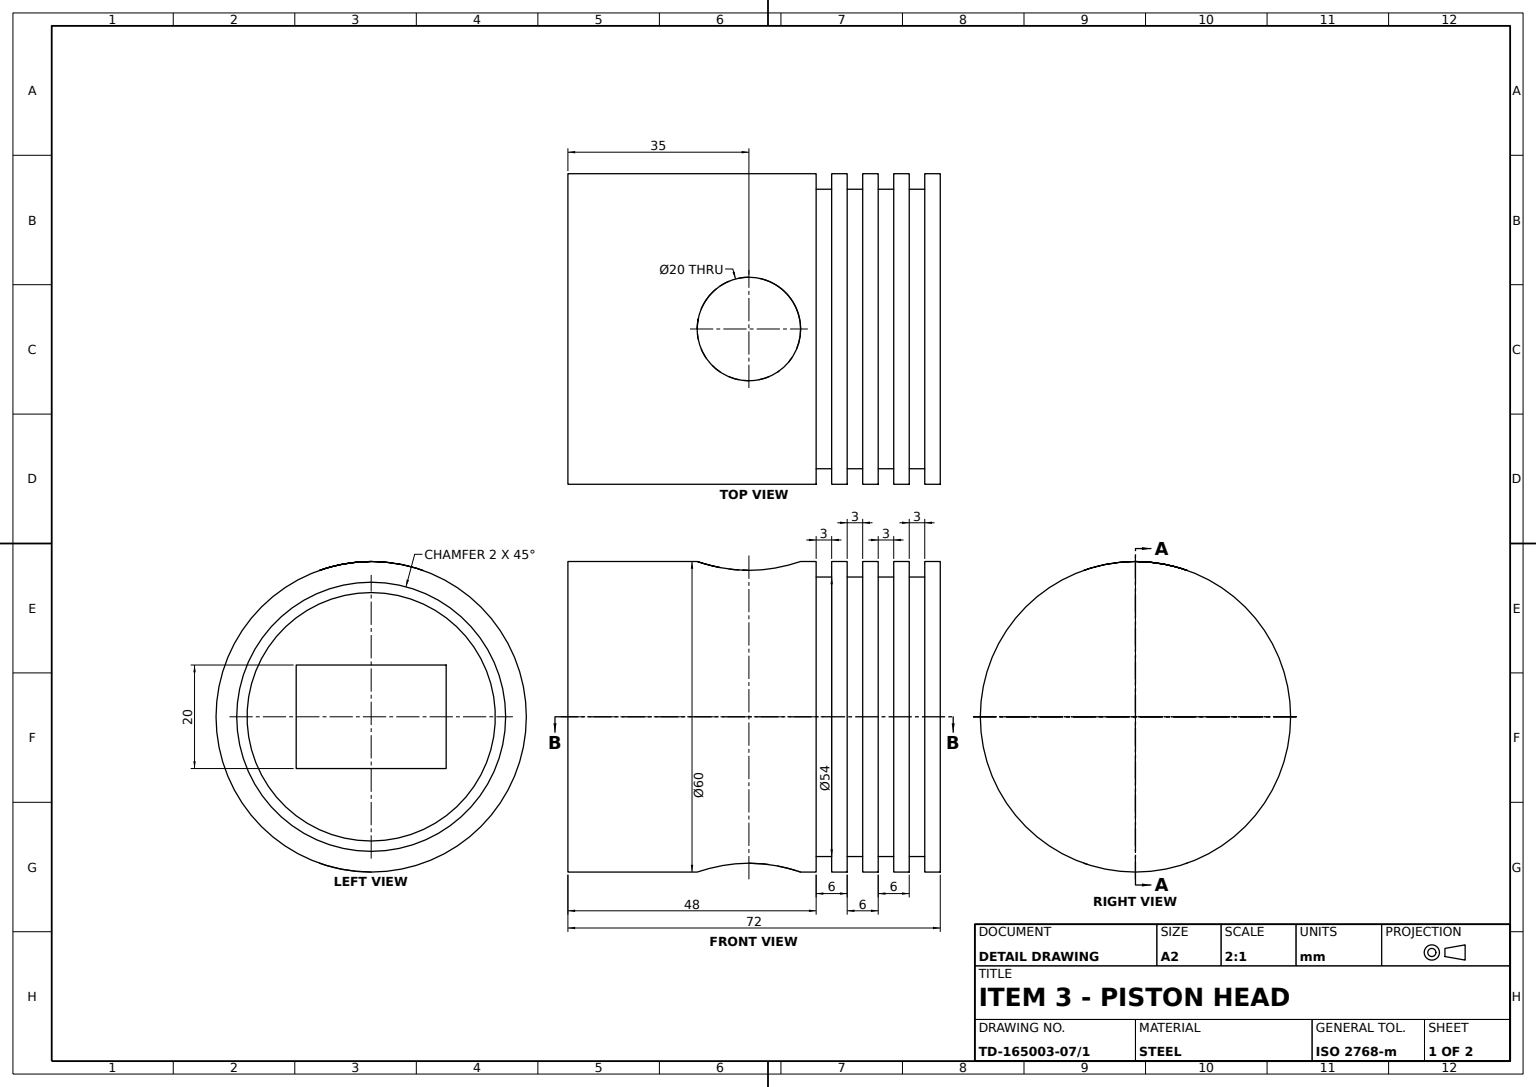
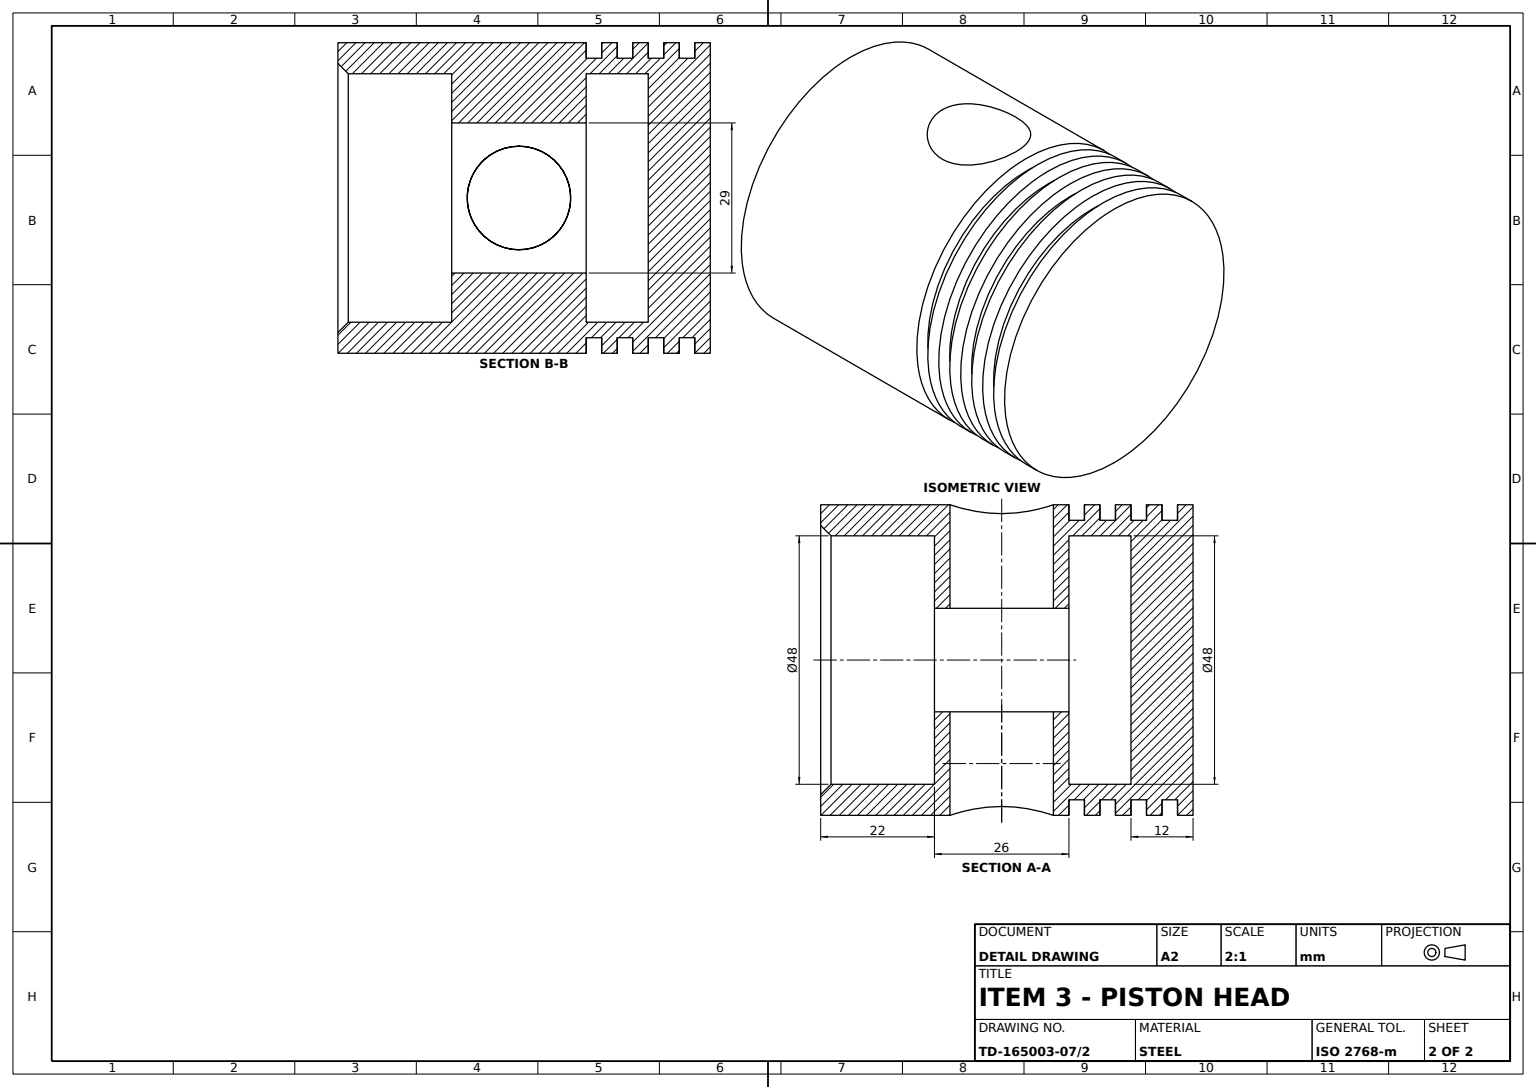
ISO-10303-21;
HEADER;
FILE_DESCRIPTION((''),'2;1');
FILE_NAME('','',(''),(''),'','','');
FILE_SCHEMA(('AUTOMOTIVE_DESIGN'));
ENDSEC;
DATA;
#1=APPLICATION_CONTEXT('');
#2=PRODUCT_CONTEXT('',#1,'mechanical');
#3=PRODUCT('','','',(#2));
#4=PRODUCT_DEFINITION_FORMATION('','',#3);
#5=PRODUCT_DEFINITION_CONTEXT('',#1,'design');
#6=PRODUCT_DEFINITION('','',#4,#5);
#7=PRODUCT_DEFINITION_SHAPE('','',#6);
#8=(LENGTH_UNIT()NAMED_UNIT(*)SI_UNIT(.MILLI.,.METRE.));
#9=(NAMED_UNIT(*)PLANE_ANGLE_UNIT()SI_UNIT($,.RADIAN.));
#10=(NAMED_UNIT(*)SI_UNIT($,.STERADIAN.)SOLID_ANGLE_UNIT());
#11=UNCERTAINTY_MEASURE_WITH_UNIT(LENGTH_MEASURE(1.E-05),#8,'distance_accuracy_value','');
#12=(GEOMETRIC_REPRESENTATION_CONTEXT(3)GLOBAL_UNCERTAINTY_ASSIGNED_CONTEXT((#11))GLOBAL_UNIT_ASSIGNED_CONTEXT((#8,#9,#10))REPRESENTATION_CONTEXT('',''));
#13=CARTESIAN_POINT('',(27.,51.,0.));
#14=VERTEX_POINT('',#13);
#15=CARTESIAN_POINT('',(27.,48.,0.));
#16=VERTEX_POINT('',#15);
#17=CARTESIAN_POINT('',(27.,60.,0.));
#18=DIRECTION('',(0.,-1.,0.));
#19=VECTOR('',#18,1000.);
#20=LINE('',#17,#19);
#21=EDGE_CURVE('',#14,#16,#20,.T.);
#22=ORIENTED_EDGE('',*,*,#21,.T.);
#23=CARTESIAN_POINT('',(-27.,48.,0.));
#24=VERTEX_POINT('',#23);
#25=CARTESIAN_POINT('',(0.,48.,0.));
#26=DIRECTION('',(1.,0.,0.));
#27=AXIS2_PLACEMENT_3D('',#25,#18,#26);
#28=CIRCLE('',#27,27.);
#29=EDGE_CURVE('',#24,#16,#28,.T.);
#30=ORIENTED_EDGE('',*,*,#29,.F.);
#31=CARTESIAN_POINT('',(-27.,51.,0.));
#32=VERTEX_POINT('',#31);
#33=CARTESIAN_POINT('',(-27.,60.,0.));
#34=LINE('',#33,#19);
#35=EDGE_CURVE('',#32,#24,#34,.T.);
#36=ORIENTED_EDGE('',*,*,#35,.F.);
#37=CARTESIAN_POINT('',(0.,51.,0.));
#38=AXIS2_PLACEMENT_3D('',#37,#18,#26);
#39=CIRCLE('',#38,27.);
#40=EDGE_CURVE('',#32,#14,#39,.T.);
#41=ORIENTED_EDGE('',*,*,#40,.T.);
#42=EDGE_LOOP('',(#22,#30,#36,#41));
#43=FACE_OUTER_BOUND('',#42,.T.);
#44=CARTESIAN_POINT('',(0.,60.,0.));
#45=AXIS2_PLACEMENT_3D('',#44,#18,#26);
#46=CYLINDRICAL_SURFACE('',#45,27.);
#47=ADVANCED_FACE('',(#43),#46,.T.);
#48=CARTESIAN_POINT('',(27.,69.,0.));
#49=VERTEX_POINT('',#48);
#50=CARTESIAN_POINT('',(-27.,69.,0.));
#51=VERTEX_POINT('',#50);
#52=CARTESIAN_POINT('',(0.,69.,0.));
#53=AXIS2_PLACEMENT_3D('',#52,#18,#26);
#54=CIRCLE('',#53,27.);
#55=EDGE_CURVE('',#49,#51,#54,.T.);
#56=ORIENTED_EDGE('',*,*,#55,.T.);
#57=CARTESIAN_POINT('',(-27.,66.,0.));
#58=VERTEX_POINT('',#57);
#59=EDGE_CURVE('',#51,#58,#34,.T.);
#60=ORIENTED_EDGE('',*,*,#59,.T.);
#61=CARTESIAN_POINT('',(27.,66.,0.));
#62=VERTEX_POINT('',#61);
#63=CARTESIAN_POINT('',(0.,66.,0.));
#64=AXIS2_PLACEMENT_3D('',#63,#18,#26);
#65=CIRCLE('',#64,27.);
#66=EDGE_CURVE('',#62,#58,#65,.T.);
#67=ORIENTED_EDGE('',*,*,#66,.F.);
#68=EDGE_CURVE('',#49,#62,#20,.T.);
#69=ORIENTED_EDGE('',*,*,#68,.F.);
#70=EDGE_LOOP('',(#56,#60,#67,#69));
#71=FACE_OUTER_BOUND('',#70,.T.);
#72=ADVANCED_FACE('',(#71),#46,.T.);
#73=CARTESIAN_POINT('',(-30.,54.,0.));
#74=VERTEX_POINT('',#73);
#75=CARTESIAN_POINT('',(-30.,51.,0.));
#76=VERTEX_POINT('',#75);
#77=CARTESIAN_POINT('',(-30.,60.,0.));
#78=LINE('',#77,#19);
#79=EDGE_CURVE('',#74,#76,#78,.T.);
#80=ORIENTED_EDGE('',*,*,#79,.T.);
#81=CARTESIAN_POINT('',(30.,51.,0.));
#82=VERTEX_POINT('',#81);
#83=CIRCLE('',#38,30.);
#84=EDGE_CURVE('',#82,#76,#83,.T.);
#85=ORIENTED_EDGE('',*,*,#84,.F.);
#86=CARTESIAN_POINT('',(30.,54.,0.));
#87=VERTEX_POINT('',#86);
#88=CARTESIAN_POINT('',(30.,60.,0.));
#89=LINE('',#88,#19);
#90=EDGE_CURVE('',#87,#82,#89,.T.);
#91=ORIENTED_EDGE('',*,*,#90,.F.);
#92=CARTESIAN_POINT('',(0.,54.,0.));
#93=AXIS2_PLACEMENT_3D('',#92,#18,#26);
#94=CIRCLE('',#93,30.);
#95=EDGE_CURVE('',#87,#74,#94,.T.);
#96=ORIENTED_EDGE('',*,*,#95,.T.);
#97=EDGE_LOOP('',(#80,#85,#91,#96));
#98=FACE_OUTER_BOUND('',#97,.T.);
#99=CYLINDRICAL_SURFACE('',#45,30.);
#100=ADVANCED_FACE('',(#98),#99,.T.);
#101=CARTESIAN_POINT('',(30.,48.,0.));
#102=VERTEX_POINT('',#101);
#103=CARTESIAN_POINT('',(-30.,48.,0.));
#104=VERTEX_POINT('',#103);
#105=CIRCLE('',#27,30.);
#106=EDGE_CURVE('',#102,#104,#105,.T.);
#107=ORIENTED_EDGE('',*,*,#106,.F.);
#108=EDGE_CURVE('',#104,#102,#105,.T.);
#109=ORIENTED_EDGE('',*,*,#108,.F.);
#110=EDGE_LOOP('',(#107,#109));
#111=FACE_OUTER_BOUND('',#110,.T.);
#112=EDGE_CURVE('',#16,#24,#28,.T.);
#113=ORIENTED_EDGE('',*,*,#112,.T.);
#114=ORIENTED_EDGE('',*,*,#29,.T.);
#115=EDGE_LOOP('',(#113,#114));
#116=FACE_BOUND('',#115,.T.);
#117=AXIS2_PLACEMENT_3D('',#103,#18,#26);
#118=PLANE('',#117);
#119=ADVANCED_FACE('',(#111,#116),#118,.F.);
#120=VERTEX_POINT('',#77);
#121=VERTEX_POINT('',#88);
#122=CIRCLE('',#45,30.);
#123=EDGE_CURVE('',#120,#121,#122,.T.);
#124=ORIENTED_EDGE('',*,*,#123,.F.);
#125=EDGE_CURVE('',#121,#120,#122,.T.);
#126=ORIENTED_EDGE('',*,*,#125,.F.);
#127=EDGE_LOOP('',(#124,#126));
#128=FACE_OUTER_BOUND('',#127,.T.);
#129=VERTEX_POINT('',#33);
#130=VERTEX_POINT('',#17);
#131=CIRCLE('',#45,27.);
#132=EDGE_CURVE('',#129,#130,#131,.T.);
#133=ORIENTED_EDGE('',*,*,#132,.T.);
#134=EDGE_CURVE('',#130,#129,#131,.T.);
#135=ORIENTED_EDGE('',*,*,#134,.T.);
#136=EDGE_LOOP('',(#133,#135));
#137=FACE_BOUND('',#136,.T.);
#138=AXIS2_PLACEMENT_3D('',#77,#18,#26);
#139=PLANE('',#138);
#140=ADVANCED_FACE('',(#128,#137),#139,.F.);
#141=CARTESIAN_POINT('',(-30.,66.,0.));
#142=VERTEX_POINT('',#141);
#143=CARTESIAN_POINT('',(30.,66.,0.));
#144=VERTEX_POINT('',#143);
#145=CIRCLE('',#64,30.);
#146=EDGE_CURVE('',#142,#144,#145,.T.);
#147=ORIENTED_EDGE('',*,*,#146,.T.);
#148=CARTESIAN_POINT('',(30.,63.,0.));
#149=VERTEX_POINT('',#148);
#150=EDGE_CURVE('',#144,#149,#89,.T.);
#151=ORIENTED_EDGE('',*,*,#150,.T.);
#152=CARTESIAN_POINT('',(-30.,63.,0.));
#153=VERTEX_POINT('',#152);
#154=CARTESIAN_POINT('',(0.,63.,0.));
#155=AXIS2_PLACEMENT_3D('',#154,#18,#26);
#156=CIRCLE('',#155,30.);
#157=EDGE_CURVE('',#153,#149,#156,.T.);
#158=ORIENTED_EDGE('',*,*,#157,.F.);
#159=EDGE_CURVE('',#142,#153,#78,.T.);
#160=ORIENTED_EDGE('',*,*,#159,.F.);
#161=EDGE_LOOP('',(#147,#151,#158,#160));
#162=FACE_OUTER_BOUND('',#161,.T.);
#163=ADVANCED_FACE('',(#162),#99,.T.);
#164=CARTESIAN_POINT('',(-27.,63.,0.));
#165=VERTEX_POINT('',#164);
#166=EDGE_CURVE('',#165,#129,#34,.T.);
#167=ORIENTED_EDGE('',*,*,#166,.F.);
#168=CARTESIAN_POINT('',(27.,63.,0.));
#169=VERTEX_POINT('',#168);
#170=CIRCLE('',#155,27.);
#171=EDGE_CURVE('',#165,#169,#170,.T.);
#172=ORIENTED_EDGE('',*,*,#171,.T.);
#173=EDGE_CURVE('',#169,#130,#20,.T.);
#174=ORIENTED_EDGE('',*,*,#173,.T.);
#175=ORIENTED_EDGE('',*,*,#132,.F.);
#176=EDGE_LOOP('',(#167,#172,#174,#175));
#177=FACE_OUTER_BOUND('',#176,.T.);
#178=ADVANCED_FACE('',(#177),#46,.T.);
#179=CARTESIAN_POINT('',(24.,2.,0.));
#180=VERTEX_POINT('',#179);
#181=CARTESIAN_POINT('',(26.,0.,0.));
#182=VERTEX_POINT('',#181);
#183=DIRECTION('',(0.707106781,-0.707106781,0.));
#184=VECTOR('',#183,1000.);
#185=LINE('',#179,#184);
#186=EDGE_CURVE('',#180,#182,#185,.T.);
#187=ORIENTED_EDGE('',*,*,#186,.F.);
#188=CARTESIAN_POINT('',(-24.,2.,0.));
#189=VERTEX_POINT('',#188);
#190=CARTESIAN_POINT('',(0.,2.,0.));
#191=DIRECTION('',(-1.,0.,0.));
#192=AXIS2_PLACEMENT_3D('',#190,#18,#191);
#193=CIRCLE('',#192,24.);
#194=EDGE_CURVE('',#189,#180,#193,.T.);
#195=ORIENTED_EDGE('',*,*,#194,.F.);
#196=CARTESIAN_POINT('',(-26.,0.,0.));
#197=VERTEX_POINT('',#196);
#198=DIRECTION('',(-0.707106781,-0.707106781,0.));
#199=VECTOR('',#198,1000.);
#200=LINE('',#188,#199);
#201=EDGE_CURVE('',#189,#197,#200,.T.);
#202=ORIENTED_EDGE('',*,*,#201,.T.);
#203=CARTESIAN_POINT('',(0.,0.,0.));
#204=DIRECTION('',(0.,1.,0.));
#205=AXIS2_PLACEMENT_3D('',#203,#204,#191);
#206=CIRCLE('',#205,26.);
#207=EDGE_CURVE('',#182,#197,#206,.T.);
#208=ORIENTED_EDGE('',*,*,#207,.F.);
#209=EDGE_LOOP('',(#187,#195,#202,#208));
#210=FACE_OUTER_BOUND('',#209,.T.);
#211=AXIS2_PLACEMENT_3D('',#190,#18,#26);
#212=CONICAL_SURFACE('',#211,24.,0.785398163);
#213=ADVANCED_FACE('',(#210),#212,.F.);
#214=CARTESIAN_POINT('',(-27.,54.,0.));
#215=VERTEX_POINT('',#214);
#216=CARTESIAN_POINT('',(27.,54.,0.));
#217=VERTEX_POINT('',#216);
#218=CIRCLE('',#93,27.);
#219=EDGE_CURVE('',#215,#217,#218,.T.);
#220=ORIENTED_EDGE('',*,*,#219,.T.);
#221=EDGE_CURVE('',#217,#215,#218,.T.);
#222=ORIENTED_EDGE('',*,*,#221,.T.);
#223=EDGE_LOOP('',(#220,#222));
#224=FACE_BOUND('',#223,.T.);
#225=ORIENTED_EDGE('',*,*,#95,.F.);
#226=EDGE_CURVE('',#74,#87,#94,.T.);
#227=ORIENTED_EDGE('',*,*,#226,.F.);
#228=EDGE_LOOP('',(#225,#227));
#229=FACE_OUTER_BOUND('',#228,.T.);
#230=AXIS2_PLACEMENT_3D('',#73,#18,#26);
#231=PLANE('',#230);
#232=ADVANCED_FACE('',(#224,#229),#231,.F.);
#233=CARTESIAN_POINT('',(30.,72.,0.));
#234=VERTEX_POINT('',#233);
#235=CARTESIAN_POINT('',(30.,69.,0.));
#236=VERTEX_POINT('',#235);
#237=EDGE_CURVE('',#234,#236,#89,.T.);
#238=ORIENTED_EDGE('',*,*,#237,.F.);
#239=CARTESIAN_POINT('',(-30.,72.,0.));
#240=VERTEX_POINT('',#239);
#241=CARTESIAN_POINT('',(0.,72.,0.));
#242=AXIS2_PLACEMENT_3D('',#241,#18,#26);
#243=CIRCLE('',#242,30.);
#244=EDGE_CURVE('',#234,#240,#243,.T.);
#245=ORIENTED_EDGE('',*,*,#244,.T.);
#246=CARTESIAN_POINT('',(-30.,69.,0.));
#247=VERTEX_POINT('',#246);
#248=EDGE_CURVE('',#240,#247,#78,.T.);
#249=ORIENTED_EDGE('',*,*,#248,.T.);
#250=CIRCLE('',#53,30.);
#251=EDGE_CURVE('',#236,#247,#250,.T.);
#252=ORIENTED_EDGE('',*,*,#251,.F.);
#253=EDGE_LOOP('',(#238,#245,#249,#252));
#254=FACE_OUTER_BOUND('',#253,.T.);
#255=ADVANCED_FACE('',(#254),#99,.T.);
#256=ORIENTED_EDGE('',*,*,#84,.T.);
#257=EDGE_CURVE('',#76,#82,#83,.T.);
#258=ORIENTED_EDGE('',*,*,#257,.T.);
#259=EDGE_LOOP('',(#256,#258));
#260=FACE_OUTER_BOUND('',#259,.T.);
#261=ORIENTED_EDGE('',*,*,#40,.F.);
#262=EDGE_CURVE('',#14,#32,#39,.T.);
#263=ORIENTED_EDGE('',*,*,#262,.F.);
#264=EDGE_LOOP('',(#261,#263));
#265=FACE_BOUND('',#264,.T.);
#266=AXIS2_PLACEMENT_3D('',#31,#204,#191);
#267=PLANE('',#266);
#268=ADVANCED_FACE('',(#260,#265),#267,.F.);
#269=ORIENTED_EDGE('',*,*,#112,.F.);
#270=ORIENTED_EDGE('',*,*,#21,.F.);
#271=ORIENTED_EDGE('',*,*,#262,.T.);
#272=ORIENTED_EDGE('',*,*,#35,.T.);
#273=EDGE_LOOP('',(#269,#270,#271,#272));
#274=FACE_OUTER_BOUND('',#273,.T.);
#275=ADVANCED_FACE('',(#274),#46,.T.);
#276=CARTESIAN_POINT('',(24.,48.,0.));
#277=VERTEX_POINT('',#276);
#278=CARTESIAN_POINT('',(-24.,48.,0.));
#279=VERTEX_POINT('',#278);
#280=CIRCLE('',#27,24.);
#281=EDGE_CURVE('',#277,#279,#280,.T.);
#282=ORIENTED_EDGE('',*,*,#281,.F.);
#283=EDGE_CURVE('',#279,#277,#280,.T.);
#284=ORIENTED_EDGE('',*,*,#283,.F.);
#285=EDGE_LOOP('',(#282,#284));
#286=FACE_OUTER_BOUND('',#285,.T.);
#287=CARTESIAN_POINT('',(-10.,48.,14.5));
#288=VERTEX_POINT('',#287);
#289=CARTESIAN_POINT('',(-10.,48.,-14.5));
#290=VERTEX_POINT('',#289);
#291=DIRECTION('',(0.,0.,-1.));
#292=VECTOR('',#291,1000.);
#293=LINE('',#289,#292);
#294=EDGE_CURVE('',#288,#290,#293,.T.);
#295=ORIENTED_EDGE('',*,*,#294,.T.);
#296=CARTESIAN_POINT('',(10.,48.,-14.5));
#297=VERTEX_POINT('',#296);
#298=VECTOR('',#26,1000.);
#299=LINE('',#289,#298);
#300=EDGE_CURVE('',#290,#297,#299,.T.);
#301=ORIENTED_EDGE('',*,*,#300,.T.);
#302=CARTESIAN_POINT('',(10.,48.,14.5));
#303=VERTEX_POINT('',#302);
#304=DIRECTION('',(0.,0.,1.));
#305=VECTOR('',#304,1000.);
#306=LINE('',#296,#305);
#307=EDGE_CURVE('',#297,#303,#306,.T.);
#308=ORIENTED_EDGE('',*,*,#307,.T.);
#309=VECTOR('',#191,1000.);
#310=LINE('',#287,#309);
#311=EDGE_CURVE('',#303,#288,#310,.T.);
#312=ORIENTED_EDGE('',*,*,#311,.T.);
#313=EDGE_LOOP('',(#295,#301,#308,#312));
#314=FACE_BOUND('',#313,.T.);
#315=AXIS2_PLACEMENT_3D('',#278,#18,#26);
#316=PLANE('',#315);
#317=ADVANCED_FACE('',(#286,#314),#316,.F.);
#318=ORIENTED_EDGE('',*,*,#311,.F.);
#319=CARTESIAN_POINT('',(10.,22.,14.5));
#320=VERTEX_POINT('',#319);
#321=LINE('',#302,#19);
#322=EDGE_CURVE('',#303,#320,#321,.T.);
#323=ORIENTED_EDGE('',*,*,#322,.T.);
#324=CARTESIAN_POINT('',(-10.,22.,14.5));
#325=VERTEX_POINT('',#324);
#326=LINE('',#324,#298);
#327=EDGE_CURVE('',#325,#320,#326,.T.);
#328=ORIENTED_EDGE('',*,*,#327,.F.);
#329=LINE('',#287,#19);
#330=EDGE_CURVE('',#288,#325,#329,.T.);
#331=ORIENTED_EDGE('',*,*,#330,.F.);
#332=EDGE_LOOP('',(#318,#323,#328,#331));
#333=FACE_OUTER_BOUND('',#332,.T.);
#334=AXIS2_PLACEMENT_3D('',#287,#304,#26);
#335=PLANE('',#334);
#336=ADVANCED_FACE('',(#333),#335,.F.);
#337=CARTESIAN_POINT('',(-28.284271,35.,10.));
#338=VERTEX_POINT('',#337);
#339=CARTESIAN_POINT('',(-30.,25.,0.));
#340=VERTEX_POINT('',#339);
#341=CARTESIAN_POINT('',(-28.284271,34.672186,10.));
#342=CARTESIAN_POINT('',(-28.289972,34.344493,9.98392));
#343=CARTESIAN_POINT('',(-28.312729,33.689353,9.919201));
#344=CARTESIAN_POINT('',(-28.329927,33.360059,9.870155));
#345=CARTESIAN_POINT('',(-28.397324,32.387225,9.675273));
#346=CARTESIAN_POINT('',(-28.462732,31.762069,9.483796));
#347=CARTESIAN_POINT('',(-28.625025,30.556004,8.982065));
#348=CARTESIAN_POINT('',(-28.722898,29.971562,8.668148));
#349=CARTESIAN_POINT('',(-28.931344,28.892387,7.94475));
#350=CARTESIAN_POINT('',(-29.042519,28.391775,7.533776));
#351=CARTESIAN_POINT('',(-29.210506,27.699053,6.841256));
#352=CARTESIAN_POINT('',(-29.266606,27.478441,6.597863));
#353=CARTESIAN_POINT('',(-29.375341,27.06588,6.095521));
#354=CARTESIAN_POINT('',(-29.428274,26.872684,5.83538));
#355=CARTESIAN_POINT('',(-29.529901,26.51207,5.297166));
#356=CARTESIAN_POINT('',(-29.578596,26.344651,5.019094));
#357=CARTESIAN_POINT('',(-29.670377,26.036018,4.444478));
#358=CARTESIAN_POINT('',(-29.713666,25.894155,4.146318));
#359=CARTESIAN_POINT('',(-29.83141,25.514703,3.234591));
#360=CARTESIAN_POINT('',(-29.893196,25.324362,2.609718));
#361=CARTESIAN_POINT('',(-29.956488,25.131116,1.646898));
#362=CARTESIAN_POINT('',(-29.972687,25.082191,1.321678));
#363=CARTESIAN_POINT('',(-29.994502,25.016459,0.662329));
#364=CARTESIAN_POINT('',(-30.,25.,0.329421));
#365=B_SPLINE_CURVE_WITH_KNOTS('',3,(#337,#341,#342,#343,#344,#345,#346,#347,#348,#349,#350,#351,#352,#353,#354,#355,#356,#357,#358,#359,#360,#361,#362,#363,#364,#339),.UNSPECIFIED.,.F.,.F.,(4,2,2,2,2,2,2,2,2,2,2,2,4),(0.031490763,0.0324745,0.033458237,0.035425711,0.037393185,0.039360659,0.040344396,0.041328133,0.04231187,0.043295607,0.045263081,0.046246818,0.047230555),.UNSPECIFIED.);
#366=EDGE_CURVE('',#338,#340,#365,.T.);
#367=ORIENTED_EDGE('',*,*,#366,.T.);
#368=CARTESIAN_POINT('',(-30.,0.,0.));
#369=VERTEX_POINT('',#368);
#370=EDGE_CURVE('',#340,#369,#78,.T.);
#371=ORIENTED_EDGE('',*,*,#370,.T.);
#372=CARTESIAN_POINT('',(30.,0.,0.));
#373=VERTEX_POINT('',#372);
#374=AXIS2_PLACEMENT_3D('',#203,#18,#26);
#375=CIRCLE('',#374,30.);
#376=EDGE_CURVE('',#373,#369,#375,.T.);
#377=ORIENTED_EDGE('',*,*,#376,.F.);
#378=CARTESIAN_POINT('',(30.,25.,0.));
#379=VERTEX_POINT('',#378);
#380=EDGE_CURVE('',#379,#373,#89,.T.);
#381=ORIENTED_EDGE('',*,*,#380,.F.);
#382=CARTESIAN_POINT('',(28.284271,35.,10.));
#383=VERTEX_POINT('',#382);
#384=CARTESIAN_POINT('',(30.,25.,0.327859));
#385=CARTESIAN_POINT('',(29.994627,25.016084,0.655616));
#386=CARTESIAN_POINT('',(29.973137,25.080833,1.310924));
#387=CARTESIAN_POINT('',(29.956884,25.12991,1.640338));
#388=CARTESIAN_POINT('',(29.893035,25.324846,2.613228));
#389=CARTESIAN_POINT('',(29.830882,25.516411,3.238598));
#390=CARTESIAN_POINT('',(29.675081,26.018498,4.445179));
#391=CARTESIAN_POINT('',(29.580407,26.332756,5.030044));
#392=CARTESIAN_POINT('',(29.376414,27.056804,6.109673));
#393=CARTESIAN_POINT('',(29.266528,27.468047,6.610295));
#394=CARTESIAN_POINT('',(29.098563,28.160664,7.302743));
#395=CARTESIAN_POINT('',(29.042133,28.404124,7.523299));
#396=CARTESIAN_POINT('',(28.932174,28.906499,7.93567));
#397=CARTESIAN_POINT('',(28.878344,29.166612,8.128741));
#398=CARTESIAN_POINT('',(28.774479,29.704689,8.489083));
#399=CARTESIAN_POINT('',(28.724442,29.982651,8.656353));
#400=CARTESIAN_POINT('',(28.629708,30.556981,8.964698));
#401=CARTESIAN_POINT('',(28.584801,30.854952,9.106416));
#402=CARTESIAN_POINT('',(28.46217,31.766195,9.485539));
#403=CARTESIAN_POINT('',(28.397157,32.390741,9.675745));
#404=CARTESIAN_POINT('',(28.330364,33.353193,9.868895));
#405=CARTESIAN_POINT('',(28.313219,33.678311,9.917805));
#406=CARTESIAN_POINT('',(28.290111,34.337515,9.983528));
#407=CARTESIAN_POINT('',(28.284271,34.670546,10.));
#408=B_SPLINE_CURVE_WITH_KNOTS('',3,(#378,#384,#385,#386,#387,#388,#389,#390,#391,#392,#393,#394,#395,#396,#397,#398,#399,#400,#401,#402,#403,#404,#405,#406,#407,#382),.UNSPECIFIED.,.F.,.F.,(4,2,2,2,2,2,2,2,2,2,2,2,4),(0.031491572,0.032475359,0.033459146,0.03542672,0.037394294,0.039361868,0.040345655,0.041329442,0.042313229,0.043297016,0.045264589,0.046248376,0.047232163),.UNSPECIFIED.);
#409=EDGE_CURVE('',#379,#383,#408,.T.);
#410=ORIENTED_EDGE('',*,*,#409,.T.);
#411=CARTESIAN_POINT('',(30.,45.,0.));
#412=VERTEX_POINT('',#411);
#413=CARTESIAN_POINT('',(28.284271,35.659008,10.));
#414=CARTESIAN_POINT('',(28.307326,36.311568,9.93549));
#415=CARTESIAN_POINT('',(28.374252,37.280808,9.741994));
#416=CARTESIAN_POINT('',(28.402148,37.603855,9.660657));
#417=CARTESIAN_POINT('',(28.46678,38.233522,9.46851));
#418=CARTESIAN_POINT('',(28.503543,38.541315,9.357638));
#419=CARTESIAN_POINT('',(28.584583,39.143348,9.107083));
#420=CARTESIAN_POINT('',(28.628862,39.437589,8.967399));
#421=CARTESIAN_POINT('',(28.723617,40.012644,8.65909));
#422=CARTESIAN_POINT('',(28.774347,40.294741,8.489579));
#423=CARTESIAN_POINT('',(28.931941,41.110823,7.942717));
#424=CARTESIAN_POINT('',(29.043198,41.610986,7.530933));
#425=CARTESIAN_POINT('',(29.209934,42.29861,6.843633));
#426=CARTESIAN_POINT('',(29.2655,42.517296,6.602838));
#427=CARTESIAN_POINT('',(29.375065,42.933138,6.096928));
#428=CARTESIAN_POINT('',(29.428617,43.12857,5.833702));
#429=CARTESIAN_POINT('',(29.581596,43.671293,5.023108));
#430=CARTESIAN_POINT('',(29.674192,43.978586,4.451282));
#431=CARTESIAN_POINT('',(29.791433,44.356484,3.544493));
#432=CARTESIAN_POINT('',(29.827069,44.469019,3.232078));
#433=CARTESIAN_POINT('',(29.888671,44.661312,2.601481));
#434=CARTESIAN_POINT('',(29.914719,44.741359,2.283241));
#435=CARTESIAN_POINT('',(29.977865,44.934141,1.319811));
#436=CARTESIAN_POINT('',(30.,45.,0.665743));
#437=B_SPLINE_CURVE_WITH_KNOTS('',3,(#382,#413,#414,#415,#416,#417,#418,#419,#420,#421,#422,#423,#424,#425,#426,#427,#428,#429,#430,#431,#432,#433,#434,#435,#436,#411),.UNSPECIFIED.,.F.,.F.,(4,2,2,2,2,2,2,2,2,2,2,2,4),(0.047232163,0.049200034,0.050183969,0.051167904,0.052151839,0.053135774,0.055103645,0.05608758,0.057071515,0.059039385,0.060023321,0.061007256,0.062975126),.UNSPECIFIED.);
#438=EDGE_CURVE('',#383,#412,#437,.T.);
#439=ORIENTED_EDGE('',*,*,#438,.T.);
#440=EDGE_CURVE('',#102,#412,#89,.T.);
#441=ORIENTED_EDGE('',*,*,#440,.F.);
#442=ORIENTED_EDGE('',*,*,#106,.T.);
#443=CARTESIAN_POINT('',(-30.,45.,0.));
#444=VERTEX_POINT('',#443);
#445=EDGE_CURVE('',#104,#444,#78,.T.);
#446=ORIENTED_EDGE('',*,*,#445,.T.);
#447=CARTESIAN_POINT('',(-30.,45.,0.328799));
#448=CARTESIAN_POINT('',(-29.994563,44.983726,0.659955));
#449=CARTESIAN_POINT('',(-29.972727,44.917931,1.320972));
#450=CARTESIAN_POINT('',(-29.956493,44.868902,1.646926));
#451=CARTESIAN_POINT('',(-29.893053,44.675199,2.611679));
#452=CARTESIAN_POINT('',(-29.831109,44.484364,3.237483));
#453=CARTESIAN_POINT('',(-29.713136,44.104119,4.150136));
#454=CARTESIAN_POINT('',(-29.669903,43.962415,4.44764));
#455=CARTESIAN_POINT('',(-29.57807,43.653551,5.022194));
#456=CARTESIAN_POINT('',(-29.529313,43.485895,5.300459));
#457=CARTESIAN_POINT('',(-29.427478,43.124442,5.839412));
#458=CARTESIAN_POINT('',(-29.374397,42.930645,6.100098));
#459=CARTESIAN_POINT('',(-29.265273,42.51639,6.603803));
#460=CARTESIAN_POINT('',(-29.209054,42.29512,6.847415));
#461=CARTESIAN_POINT('',(-29.041638,41.604271,7.537049));
#462=CARTESIAN_POINT('',(-28.930641,41.104319,7.947302));
#463=CARTESIAN_POINT('',(-28.722184,40.024398,8.67051));
#464=CARTESIAN_POINT('',(-28.624378,39.439648,8.984102));
#465=CARTESIAN_POINT('',(-28.462572,38.236279,9.484253));
#466=CARTESIAN_POINT('',(-28.397341,37.612576,9.675219));
#467=CARTESIAN_POINT('',(-28.33006,36.642093,9.869771));
#468=CARTESIAN_POINT('',(-28.312784,36.311953,9.919046));
#469=CARTESIAN_POINT('',(-28.289973,35.655792,9.983918));
#470=CARTESIAN_POINT('',(-28.284271,35.327835,10.));
#471=B_SPLINE_CURVE_WITH_KNOTS('',3,(#443,#447,#448,#449,#450,#451,#452,#453,#454,#455,#456,#457,#458,#459,#460,#461,#462,#463,#464,#465,#466,#467,#468,#469,#470,#337),.UNSPECIFIED.,.F.,.F.,(4,2,2,2,2,2,2,2,2,2,2,2,4),(0.015749947,0.016733748,0.017717549,0.019685151,0.020668952,0.021652753,0.022636554,0.023620355,0.025587957,0.027555559,0.029523161,0.030506962,0.031490763),.UNSPECIFIED.);
#472=EDGE_CURVE('',#444,#338,#471,.T.);
#473=ORIENTED_EDGE('',*,*,#472,.T.);
#474=EDGE_LOOP('',(#367,#371,#377,#381,#410,#439,#441,#442,#446,#473));
#475=FACE_OUTER_BOUND('',#474,.T.);
#476=ADVANCED_FACE('',(#475),#99,.T.);
#477=ORIENTED_EDGE('',*,*,#221,.F.);
#478=CARTESIAN_POINT('',(27.,57.,0.));
#479=VERTEX_POINT('',#478);
#480=EDGE_CURVE('',#479,#217,#20,.T.);
#481=ORIENTED_EDGE('',*,*,#480,.F.);
#482=CARTESIAN_POINT('',(-27.,57.,0.));
#483=VERTEX_POINT('',#482);
#484=CARTESIAN_POINT('',(0.,57.,0.));
#485=AXIS2_PLACEMENT_3D('',#484,#18,#26);
#486=CIRCLE('',#485,27.);
#487=EDGE_CURVE('',#479,#483,#486,.T.);
#488=ORIENTED_EDGE('',*,*,#487,.T.);
#489=EDGE_CURVE('',#483,#215,#34,.T.);
#490=ORIENTED_EDGE('',*,*,#489,.T.);
#491=EDGE_LOOP('',(#477,#481,#488,#490));
#492=FACE_OUTER_BOUND('',#491,.T.);
#493=ADVANCED_FACE('',(#492),#46,.T.);
#494=CARTESIAN_POINT('',(24.,60.,0.));
#495=VERTEX_POINT('',#494);
#496=CARTESIAN_POINT('',(-24.,60.,0.));
#497=VERTEX_POINT('',#496);
#498=CIRCLE('',#45,24.);
#499=EDGE_CURVE('',#495,#497,#498,.T.);
#500=ORIENTED_EDGE('',*,*,#499,.T.);
#501=EDGE_CURVE('',#497,#495,#498,.T.);
#502=ORIENTED_EDGE('',*,*,#501,.T.);
#503=EDGE_LOOP('',(#500,#502));
#504=FACE_OUTER_BOUND('',#503,.T.);
#505=AXIS2_PLACEMENT_3D('',#496,#204,#191);
#506=PLANE('',#505);
#507=ADVANCED_FACE('',(#504),#506,.F.);
#508=CARTESIAN_POINT('',(-10.,22.,-14.5));
#509=VERTEX_POINT('',#508);
#510=LINE('',#289,#19);
#511=EDGE_CURVE('',#290,#509,#510,.T.);
#512=ORIENTED_EDGE('',*,*,#511,.T.);
#513=CARTESIAN_POINT('',(10.,22.,-14.5));
#514=VERTEX_POINT('',#513);
#515=LINE('',#508,#309);
#516=EDGE_CURVE('',#514,#509,#515,.T.);
#517=ORIENTED_EDGE('',*,*,#516,.F.);
#518=LINE('',#296,#19);
#519=EDGE_CURVE('',#297,#514,#518,.T.);
#520=ORIENTED_EDGE('',*,*,#519,.F.);
#521=ORIENTED_EDGE('',*,*,#300,.F.);
#522=EDGE_LOOP('',(#512,#517,#520,#521));
#523=FACE_OUTER_BOUND('',#522,.T.);
#524=AXIS2_PLACEMENT_3D('',#289,#291,#191);
#525=PLANE('',#524);
#526=ADVANCED_FACE('',(#523),#525,.F.);
#527=CARTESIAN_POINT('',(24.,22.,0.));
#528=VERTEX_POINT('',#527);
#529=CARTESIAN_POINT('',(-24.,22.,0.));
#530=VERTEX_POINT('',#529);
#531=CARTESIAN_POINT('',(0.,22.,0.));
#532=AXIS2_PLACEMENT_3D('',#531,#18,#26);
#533=CIRCLE('',#532,24.);
#534=EDGE_CURVE('',#528,#530,#533,.T.);
#535=ORIENTED_EDGE('',*,*,#534,.T.);
#536=EDGE_CURVE('',#530,#528,#533,.T.);
#537=ORIENTED_EDGE('',*,*,#536,.T.);
#538=EDGE_LOOP('',(#535,#537));
#539=FACE_OUTER_BOUND('',#538,.T.);
#540=CARTESIAN_POINT('',(10.,22.,0.));
#541=LINE('',#540,#292);
#542=EDGE_CURVE('',#320,#514,#541,.T.);
#543=ORIENTED_EDGE('',*,*,#542,.T.);
#544=ORIENTED_EDGE('',*,*,#516,.T.);
#545=CARTESIAN_POINT('',(-10.,22.,0.));
#546=LINE('',#545,#305);
#547=EDGE_CURVE('',#509,#325,#546,.T.);
#548=ORIENTED_EDGE('',*,*,#547,.T.);
#549=ORIENTED_EDGE('',*,*,#327,.T.);
#550=EDGE_LOOP('',(#543,#544,#548,#549));
#551=FACE_BOUND('',#550,.T.);
#552=AXIS2_PLACEMENT_3D('',#545,#204,#191);
#553=PLANE('',#552);
#554=ADVANCED_FACE('',(#539,#551),#553,.F.);
#555=EDGE_CURVE('',#483,#479,#486,.T.);
#556=ORIENTED_EDGE('',*,*,#555,.F.);
#557=ORIENTED_EDGE('',*,*,#487,.F.);
#558=EDGE_LOOP('',(#556,#557));
#559=FACE_BOUND('',#558,.T.);
#560=CARTESIAN_POINT('',(30.,57.,0.));
#561=VERTEX_POINT('',#560);
#562=CARTESIAN_POINT('',(-30.,57.,0.));
#563=VERTEX_POINT('',#562);
#564=CIRCLE('',#485,30.);
#565=EDGE_CURVE('',#561,#563,#564,.T.);
#566=ORIENTED_EDGE('',*,*,#565,.T.);
#567=EDGE_CURVE('',#563,#561,#564,.T.);
#568=ORIENTED_EDGE('',*,*,#567,.T.);
#569=EDGE_LOOP('',(#566,#568));
#570=FACE_OUTER_BOUND('',#569,.T.);
#571=AXIS2_PLACEMENT_3D('',#482,#204,#191);
#572=PLANE('',#571);
#573=ADVANCED_FACE('',(#559,#570),#572,.F.);
#574=CARTESIAN_POINT('',(10.,35.,10.));
#575=VERTEX_POINT('',#574);
#576=CARTESIAN_POINT('',(-66.,35.,10.));
#577=LINE('',#576,#298);
#578=EDGE_CURVE('',#575,#383,#577,.T.);
#579=ORIENTED_EDGE('',*,*,#578,.T.);
#580=ORIENTED_EDGE('',*,*,#409,.F.);
#581=CARTESIAN_POINT('',(28.284271,35.,-10.));
#582=VERTEX_POINT('',#581);
#583=CARTESIAN_POINT('',(28.284271,34.671279,-10.));
#584=CARTESIAN_POINT('',(28.290035,34.340297,-9.983744));
#585=CARTESIAN_POINT('',(28.313167,33.679179,-9.917953));
#586=CARTESIAN_POINT('',(28.330354,33.353226,-9.868926));
#587=CARTESIAN_POINT('',(28.397321,32.3886,-9.675268));
#588=CARTESIAN_POINT('',(28.462516,31.76304,-9.484518));
#589=CARTESIAN_POINT('',(28.585393,30.850845,-9.10456));
#590=CARTESIAN_POINT('',(28.630237,30.553579,-8.963012));
#591=CARTESIAN_POINT('',(28.72502,29.979348,-8.654438));
#592=CARTESIAN_POINT('',(28.775117,29.701207,-8.48693));
#593=CARTESIAN_POINT('',(28.879189,29.162414,-8.125748));
#594=CARTESIAN_POINT('',(28.933166,28.901762,-7.932074));
#595=CARTESIAN_POINT('',(29.043512,28.398032,-7.518));
#596=CARTESIAN_POINT('',(29.100035,28.154432,-7.296851));
#597=CARTESIAN_POINT('',(29.267404,27.464758,-6.60632));
#598=CARTESIAN_POINT('',(29.377101,27.054268,-6.106397));
#599=CARTESIAN_POINT('',(29.581082,26.330455,-5.026104));
#600=CARTESIAN_POINT('',(29.675682,26.01653,-4.440983));
#601=CARTESIAN_POINT('',(29.831033,25.515954,-3.236962));
#602=CARTESIAN_POINT('',(29.893032,25.324858,-2.612921));
#603=CARTESIAN_POINT('',(29.956781,25.130224,-1.642089));
#604=CARTESIAN_POINT('',(29.973096,25.080957,-1.311971));
#605=CARTESIAN_POINT('',(29.994627,25.016085,-0.655831));
#606=CARTESIAN_POINT('',(30.,25.,-0.327864));
#607=B_SPLINE_CURVE_WITH_KNOTS('',3,(#581,#583,#584,#585,#586,#587,#588,#589,#590,#591,#592,#593,#594,#595,#596,#597,#598,#599,#600,#601,#602,#603,#604,#605,#606,#378),.UNSPECIFIED.,.F.,.F.,(4,2,2,2,2,2,2,2,2,2,2,2,4),(0.015750734,0.016734537,0.017718339,0.019685944,0.020669746,0.021653548,0.022637351,0.023621153,0.025588758,0.027556363,0.029523967,0.03050777,0.031491572),.UNSPECIFIED.);
#608=EDGE_CURVE('',#582,#379,#607,.T.);
#609=ORIENTED_EDGE('',*,*,#608,.F.);
#610=CARTESIAN_POINT('',(10.,35.,-10.));
#611=VERTEX_POINT('',#610);
#612=CARTESIAN_POINT('',(-66.,35.,-10.));
#613=LINE('',#612,#298);
#614=EDGE_CURVE('',#611,#582,#613,.T.);
#615=ORIENTED_EDGE('',*,*,#614,.F.);
#616=CARTESIAN_POINT('',(10.,35.,0.));
#617=AXIS2_PLACEMENT_3D('',#616,#191,#204);
#618=CIRCLE('',#617,10.);
#619=EDGE_CURVE('',#611,#575,#618,.T.);
#620=ORIENTED_EDGE('',*,*,#619,.T.);
#621=EDGE_LOOP('',(#579,#580,#609,#615,#620));
#622=FACE_OUTER_BOUND('',#621,.T.);
#623=CARTESIAN_POINT('',(-66.,35.,0.));
#624=AXIS2_PLACEMENT_3D('',#623,#26,#291);
#625=CYLINDRICAL_SURFACE('',#624,10.);
#626=ADVANCED_FACE('',(#622),#625,.F.);
#627=EDGE_CURVE('',#197,#182,#206,.T.);
#628=ORIENTED_EDGE('',*,*,#627,.F.);
#629=ORIENTED_EDGE('',*,*,#201,.F.);
#630=EDGE_CURVE('',#180,#189,#193,.T.);
#631=ORIENTED_EDGE('',*,*,#630,.F.);
#632=ORIENTED_EDGE('',*,*,#186,.T.);
#633=EDGE_LOOP('',(#628,#629,#631,#632));
#634=FACE_OUTER_BOUND('',#633,.T.);
#635=ADVANCED_FACE('',(#634),#212,.F.);
#636=CARTESIAN_POINT('',(-10.,35.,10.));
#637=VERTEX_POINT('',#636);
#638=CARTESIAN_POINT('',(-10.,35.,-10.));
#639=VERTEX_POINT('',#638);
#640=CARTESIAN_POINT('',(-10.,35.,0.));
#641=AXIS2_PLACEMENT_3D('',#640,#26,#18);
#642=CIRCLE('',#641,10.);
#643=EDGE_CURVE('',#637,#639,#642,.T.);
#644=ORIENTED_EDGE('',*,*,#643,.F.);
#645=EDGE_CURVE('',#639,#637,#642,.T.);
#646=ORIENTED_EDGE('',*,*,#645,.F.);
#647=EDGE_LOOP('',(#644,#646));
#648=FACE_BOUND('',#647,.T.);
#649=ORIENTED_EDGE('',*,*,#511,.F.);
#650=ORIENTED_EDGE('',*,*,#294,.F.);
#651=ORIENTED_EDGE('',*,*,#330,.T.);
#652=ORIENTED_EDGE('',*,*,#547,.F.);
#653=EDGE_LOOP('',(#649,#650,#651,#652));
#654=FACE_OUTER_BOUND('',#653,.T.);
#655=AXIS2_PLACEMENT_3D('',#289,#191,#18);
#656=PLANE('',#655);
#657=ADVANCED_FACE('',(#648,#654),#656,.F.);
#658=ORIENTED_EDGE('',*,*,#257,.F.);
#659=ORIENTED_EDGE('',*,*,#79,.F.);
#660=ORIENTED_EDGE('',*,*,#226,.T.);
#661=ORIENTED_EDGE('',*,*,#90,.T.);
#662=EDGE_LOOP('',(#658,#659,#660,#661));
#663=FACE_OUTER_BOUND('',#662,.T.);
#664=ADVANCED_FACE('',(#663),#99,.T.);
#665=ORIENTED_EDGE('',*,*,#68,.T.);
#666=EDGE_CURVE('',#58,#62,#65,.T.);
#667=ORIENTED_EDGE('',*,*,#666,.F.);
#668=ORIENTED_EDGE('',*,*,#59,.F.);
#669=EDGE_CURVE('',#51,#49,#54,.T.);
#670=ORIENTED_EDGE('',*,*,#669,.T.);
#671=EDGE_LOOP('',(#665,#667,#668,#670));
#672=FACE_OUTER_BOUND('',#671,.T.);
#673=ADVANCED_FACE('',(#672),#46,.T.);
#674=ORIENTED_EDGE('',*,*,#630,.T.);
#675=LINE('',#496,#19);
#676=EDGE_CURVE('',#530,#189,#675,.T.);
#677=ORIENTED_EDGE('',*,*,#676,.F.);
#678=ORIENTED_EDGE('',*,*,#534,.F.);
#679=LINE('',#494,#19);
#680=EDGE_CURVE('',#528,#180,#679,.T.);
#681=ORIENTED_EDGE('',*,*,#680,.T.);
#682=EDGE_LOOP('',(#674,#677,#678,#681));
#683=FACE_OUTER_BOUND('',#682,.T.);
#684=CYLINDRICAL_SURFACE('',#45,24.);
#685=ADVANCED_FACE('',(#683),#684,.F.);
#686=EDGE_CURVE('',#240,#234,#243,.T.);
#687=ORIENTED_EDGE('',*,*,#686,.F.);
#688=ORIENTED_EDGE('',*,*,#244,.F.);
#689=EDGE_LOOP('',(#687,#688));
#690=FACE_OUTER_BOUND('',#689,.T.);
#691=AXIS2_PLACEMENT_3D('',#239,#18,#26);
#692=PLANE('',#691);
#693=ADVANCED_FACE('',(#690),#692,.F.);
#694=ORIENTED_EDGE('',*,*,#645,.T.);
#695=EDGE_CURVE('',#338,#637,#577,.T.);
#696=ORIENTED_EDGE('',*,*,#695,.F.);
#697=ORIENTED_EDGE('',*,*,#472,.F.);
#698=CARTESIAN_POINT('',(-28.284271,35.,-10.));
#699=VERTEX_POINT('',#698);
#700=CARTESIAN_POINT('',(-28.284271,35.666104,-10.));
#701=CARTESIAN_POINT('',(-28.307804,36.320039,-9.934121));
#702=CARTESIAN_POINT('',(-28.374506,37.283693,-9.741255));
#703=CARTESIAN_POINT('',(-28.401973,37.602017,-9.661172));
#704=CARTESIAN_POINT('',(-28.466693,38.232808,-9.468774));
#705=CARTESIAN_POINT('',(-28.503971,38.544856,-9.356344));
#706=CARTESIAN_POINT('',(-28.626152,39.45143,-8.978502));
#707=CARTESIAN_POINT('',(-28.722074,40.023954,-8.670935));
#708=CARTESIAN_POINT('',(-28.878975,40.836594,-8.126529));
#709=CARTESIAN_POINT('',(-28.933742,41.100971,-7.929981));
#710=CARTESIAN_POINT('',(-29.044179,41.604904,-7.51543));
#711=CARTESIAN_POINT('',(-29.099936,41.84511,-7.29721));
#712=CARTESIAN_POINT('',(-29.266485,42.531548,-6.610217));
#713=CARTESIAN_POINT('',(-29.376582,42.943971,-6.109463));
#714=CARTESIAN_POINT('',(-29.582771,43.675453,-5.016845));
#715=CARTESIAN_POINT('',(-29.675435,43.982651,-4.442525));
#716=CARTESIAN_POINT('',(-29.791867,44.357858,-3.540693));
#717=CARTESIAN_POINT('',(-29.826935,44.468596,-3.233242));
#718=CARTESIAN_POINT('',(-29.888432,44.660572,-2.604132));
#719=CARTESIAN_POINT('',(-29.91493,44.74201,-2.280798));
#720=CARTESIAN_POINT('',(-29.978376,44.93569,-1.310432));
#721=CARTESIAN_POINT('',(-30.,45.,-0.65798));
#722=B_SPLINE_CURVE_WITH_KNOTS('',3,(#698,#700,#701,#702,#703,#704,#705,#706,#707,#708,#709,#710,#711,#712,#713,#714,#715,#716,#717,#718,#719,#720,#721,#443),.UNSPECIFIED.,.F.,.F.,(4,2,2,2,2,2,2,2,2,2,2,4),(0.,0.001968743,0.002953115,0.003937487,0.00590623,0.006890602,0.007874973,0.009843717,0.01181246,0.012796832,0.013781204,0.015749947),.UNSPECIFIED.);
#723=EDGE_CURVE('',#699,#444,#722,.T.);
#724=ORIENTED_EDGE('',*,*,#723,.F.);
#725=EDGE_CURVE('',#699,#639,#613,.T.);
#726=ORIENTED_EDGE('',*,*,#725,.T.);
#727=EDGE_LOOP('',(#694,#696,#697,#724,#726));
#728=FACE_OUTER_BOUND('',#727,.T.);
#729=ADVANCED_FACE('',(#728),#625,.F.);
#730=EDGE_CURVE('',#149,#153,#156,.T.);
#731=ORIENTED_EDGE('',*,*,#730,.F.);
#732=ORIENTED_EDGE('',*,*,#150,.F.);
#733=EDGE_CURVE('',#144,#142,#145,.T.);
#734=ORIENTED_EDGE('',*,*,#733,.T.);
#735=ORIENTED_EDGE('',*,*,#159,.T.);
#736=EDGE_LOOP('',(#731,#732,#734,#735));
#737=FACE_OUTER_BOUND('',#736,.T.);
#738=ADVANCED_FACE('',(#737),#99,.T.);
#739=ORIENTED_EDGE('',*,*,#55,.F.);
#740=ORIENTED_EDGE('',*,*,#669,.F.);
#741=EDGE_LOOP('',(#739,#740));
#742=FACE_BOUND('',#741,.T.);
#743=EDGE_CURVE('',#247,#236,#250,.T.);
#744=ORIENTED_EDGE('',*,*,#743,.T.);
#745=ORIENTED_EDGE('',*,*,#251,.T.);
#746=EDGE_LOOP('',(#744,#745));
#747=FACE_OUTER_BOUND('',#746,.T.);
#748=AXIS2_PLACEMENT_3D('',#50,#204,#191);
#749=PLANE('',#748);
#750=ADVANCED_FACE('',(#742,#747),#749,.F.);
#751=ORIENTED_EDGE('',*,*,#578,.F.);
#752=EDGE_CURVE('',#575,#611,#618,.T.);
#753=ORIENTED_EDGE('',*,*,#752,.T.);
#754=ORIENTED_EDGE('',*,*,#614,.T.);
#755=CARTESIAN_POINT('',(30.,45.,-0.666071));
#756=CARTESIAN_POINT('',(29.97786,44.934125,-1.320094));
#757=CARTESIAN_POINT('',(29.914662,44.741186,-2.284001));
#758=CARTESIAN_POINT('',(29.888591,44.661065,-2.602429));
#759=CARTESIAN_POINT('',(29.826922,44.468558,-3.233454));
#760=CARTESIAN_POINT('',(29.791291,44.356033,-3.545696));
#761=CARTESIAN_POINT('',(29.673969,43.977855,-4.452794));
#762=CARTESIAN_POINT('',(29.5812,43.669994,-5.025611));
#763=CARTESIAN_POINT('',(29.427682,43.125198,-5.838455));
#764=CARTESIAN_POINT('',(29.373819,42.928513,-6.102888));
#765=CARTESIAN_POINT('',(29.264561,42.513626,-6.606964));
#766=CARTESIAN_POINT('',(29.209101,42.295271,-6.847178));
#767=CARTESIAN_POINT('',(29.042524,41.60801,-7.53349));
#768=CARTESIAN_POINT('',(28.931154,41.107268,-7.945624));
#769=CARTESIAN_POINT('',(28.720461,40.015175,-8.676387));
#770=CARTESIAN_POINT('',(28.624615,39.441075,-8.98334));
#771=CARTESIAN_POINT('',(28.50335,38.53972,-9.358219));
#772=CARTESIAN_POINT('',(28.466661,38.23243,-9.468867));
#773=CARTESIAN_POINT('',(28.40213,37.603614,-9.660706));
#774=CARTESIAN_POINT('',(28.374214,37.280373,-9.742107));
#775=CARTESIAN_POINT('',(28.307247,36.310181,-9.935715));
#776=CARTESIAN_POINT('',(28.284271,35.657855,-10.));
#777=B_SPLINE_CURVE_WITH_KNOTS('',3,(#411,#755,#756,#757,#758,#759,#760,#761,#762,#763,#764,#765,#766,#767,#768,#769,#770,#771,#772,#773,#774,#775,#776,#581),.UNSPECIFIED.,.F.,.F.,(4,2,2,2,2,2,2,2,2,2,2,4),(0.,0.001968842,0.002953263,0.003937684,0.005906525,0.006890946,0.007875367,0.009844209,0.011813051,0.012797472,0.013781892,0.015750734),.UNSPECIFIED.);
#778=EDGE_CURVE('',#412,#582,#777,.T.);
#779=ORIENTED_EDGE('',*,*,#778,.F.);
#780=ORIENTED_EDGE('',*,*,#438,.F.);
#781=EDGE_LOOP('',(#751,#753,#754,#779,#780));
#782=FACE_OUTER_BOUND('',#781,.T.);
#783=ADVANCED_FACE('',(#782),#625,.F.);
#784=ORIENTED_EDGE('',*,*,#666,.T.);
#785=ORIENTED_EDGE('',*,*,#66,.T.);
#786=EDGE_LOOP('',(#784,#785));
#787=FACE_BOUND('',#786,.T.);
#788=ORIENTED_EDGE('',*,*,#146,.F.);
#789=ORIENTED_EDGE('',*,*,#733,.F.);
#790=EDGE_LOOP('',(#788,#789));
#791=FACE_OUTER_BOUND('',#790,.T.);
#792=AXIS2_PLACEMENT_3D('',#141,#18,#26);
#793=PLANE('',#792);
#794=ADVANCED_FACE('',(#787,#791),#793,.F.);
#795=EDGE_CURVE('',#120,#563,#78,.T.);
#796=ORIENTED_EDGE('',*,*,#795,.T.);
#797=ORIENTED_EDGE('',*,*,#565,.F.);
#798=EDGE_CURVE('',#121,#561,#89,.T.);
#799=ORIENTED_EDGE('',*,*,#798,.F.);
#800=ORIENTED_EDGE('',*,*,#125,.T.);
#801=EDGE_LOOP('',(#796,#797,#799,#800));
#802=FACE_OUTER_BOUND('',#801,.T.);
#803=ADVANCED_FACE('',(#802),#99,.T.);
#804=ORIENTED_EDGE('',*,*,#134,.F.);
#805=ORIENTED_EDGE('',*,*,#173,.F.);
#806=EDGE_CURVE('',#169,#165,#170,.T.);
#807=ORIENTED_EDGE('',*,*,#806,.T.);
#808=ORIENTED_EDGE('',*,*,#166,.T.);
#809=EDGE_LOOP('',(#804,#805,#807,#808));
#810=FACE_OUTER_BOUND('',#809,.T.);
#811=ADVANCED_FACE('',(#810),#46,.T.);
#812=ORIENTED_EDGE('',*,*,#778,.T.);
#813=ORIENTED_EDGE('',*,*,#608,.T.);
#814=ORIENTED_EDGE('',*,*,#380,.T.);
#815=EDGE_CURVE('',#369,#373,#375,.T.);
#816=ORIENTED_EDGE('',*,*,#815,.F.);
#817=ORIENTED_EDGE('',*,*,#370,.F.);
#818=CARTESIAN_POINT('',(-30.,25.,-0.658964));
#819=CARTESIAN_POINT('',(-29.978313,25.064503,-1.311615));
#820=CARTESIAN_POINT('',(-29.914899,25.258084,-2.28116));
#821=CARTESIAN_POINT('',(-29.88842,25.339465,-2.60432));
#822=CARTESIAN_POINT('',(-29.826836,25.531715,-3.234193));
#823=CARTESIAN_POINT('',(-29.791705,25.642657,-3.542108));
#824=CARTESIAN_POINT('',(-29.713907,25.893385,-4.144389));
#825=CARTESIAN_POINT('',(-29.671237,26.033172,-4.438754));
#826=CARTESIAN_POINT('',(-29.579458,26.341707,-5.01403));
#827=CARTESIAN_POINT('',(-29.530104,26.51132,-5.296196));
#828=CARTESIAN_POINT('',(-29.375855,27.058749,-6.11278));
#829=CARTESIAN_POINT('',(-29.265858,27.470848,-6.613012));
#830=CARTESIAN_POINT('',(-29.099129,28.15831,-7.300431));
#831=CARTESIAN_POINT('',(-29.043259,28.399108,-7.518999));
#832=CARTESIAN_POINT('',(-28.932498,28.904892,-7.934531));
#833=CARTESIAN_POINT('',(-28.87803,29.168116,-8.12987));
#834=CARTESIAN_POINT('',(-28.721674,29.978489,-8.672198));
#835=CARTESIAN_POINT('',(-28.625931,30.550018,-8.979201));
#836=CARTESIAN_POINT('',(-28.50383,31.456287,-9.356773));
#837=CARTESIAN_POINT('',(-28.466545,31.768517,-9.469218));
#838=CARTESIAN_POINT('',(-28.401892,32.398888,-9.661407));
#839=CARTESIAN_POINT('',(-28.374449,32.717028,-9.741419));
#840=CARTESIAN_POINT('',(-28.307799,33.680218,-9.934134));
#841=CARTESIAN_POINT('',(-28.284271,34.334202,-10.));
#842=B_SPLINE_CURVE_WITH_KNOTS('',3,(#339,#818,#819,#820,#821,#822,#823,#824,#825,#826,#827,#828,#829,#830,#831,#832,#833,#834,#835,#836,#837,#838,#839,#840,#841,#698),.UNSPECIFIED.,.F.,.F.,(4,2,2,2,2,2,2,2,2,2,2,2,4),(0.047230555,0.049198395,0.050182315,0.051166235,0.052150155,0.053134075,0.055101915,0.056085835,0.057069755,0.059037595,0.060021515,0.061005435,0.062973275),.UNSPECIFIED.);
#843=EDGE_CURVE('',#340,#699,#842,.T.);
#844=ORIENTED_EDGE('',*,*,#843,.T.);
#845=ORIENTED_EDGE('',*,*,#723,.T.);
#846=ORIENTED_EDGE('',*,*,#445,.F.);
#847=ORIENTED_EDGE('',*,*,#108,.T.);
#848=ORIENTED_EDGE('',*,*,#440,.T.);
#849=EDGE_LOOP('',(#812,#813,#814,#816,#817,#844,#845,#846,#847,#848));
#850=FACE_OUTER_BOUND('',#849,.T.);
#851=ADVANCED_FACE('',(#850),#99,.T.);
#852=ORIENTED_EDGE('',*,*,#730,.T.);
#853=ORIENTED_EDGE('',*,*,#157,.T.);
#854=EDGE_LOOP('',(#852,#853));
#855=FACE_OUTER_BOUND('',#854,.T.);
#856=ORIENTED_EDGE('',*,*,#171,.F.);
#857=ORIENTED_EDGE('',*,*,#806,.F.);
#858=EDGE_LOOP('',(#856,#857));
#859=FACE_BOUND('',#858,.T.);
#860=AXIS2_PLACEMENT_3D('',#164,#204,#191);
#861=PLANE('',#860);
#862=ADVANCED_FACE('',(#855,#859),#861,.F.);
#863=ORIENTED_EDGE('',*,*,#489,.F.);
#864=ORIENTED_EDGE('',*,*,#555,.T.);
#865=ORIENTED_EDGE('',*,*,#480,.T.);
#866=ORIENTED_EDGE('',*,*,#219,.F.);
#867=EDGE_LOOP('',(#863,#864,#865,#866));
#868=FACE_OUTER_BOUND('',#867,.T.);
#869=ADVANCED_FACE('',(#868),#46,.T.);
#870=EDGE_CURVE('',#497,#279,#675,.T.);
#871=ORIENTED_EDGE('',*,*,#870,.F.);
#872=ORIENTED_EDGE('',*,*,#499,.F.);
#873=EDGE_CURVE('',#495,#277,#679,.T.);
#874=ORIENTED_EDGE('',*,*,#873,.T.);
#875=ORIENTED_EDGE('',*,*,#281,.T.);
#876=EDGE_LOOP('',(#871,#872,#874,#875));
#877=FACE_OUTER_BOUND('',#876,.T.);
#878=ADVANCED_FACE('',(#877),#684,.F.);
#879=ORIENTED_EDGE('',*,*,#795,.F.);
#880=ORIENTED_EDGE('',*,*,#123,.T.);
#881=ORIENTED_EDGE('',*,*,#798,.T.);
#882=ORIENTED_EDGE('',*,*,#567,.F.);
#883=EDGE_LOOP('',(#879,#880,#881,#882));
#884=FACE_OUTER_BOUND('',#883,.T.);
#885=ADVANCED_FACE('',(#884),#99,.T.);
#886=ORIENTED_EDGE('',*,*,#501,.F.);
#887=ORIENTED_EDGE('',*,*,#870,.T.);
#888=ORIENTED_EDGE('',*,*,#283,.T.);
#889=ORIENTED_EDGE('',*,*,#873,.F.);
#890=EDGE_LOOP('',(#886,#887,#888,#889));
#891=FACE_OUTER_BOUND('',#890,.T.);
#892=ADVANCED_FACE('',(#891),#684,.F.);
#893=ORIENTED_EDGE('',*,*,#843,.F.);
#894=ORIENTED_EDGE('',*,*,#366,.F.);
#895=ORIENTED_EDGE('',*,*,#695,.T.);
#896=ORIENTED_EDGE('',*,*,#643,.T.);
#897=ORIENTED_EDGE('',*,*,#725,.F.);
#898=EDGE_LOOP('',(#893,#894,#895,#896,#897));
#899=FACE_OUTER_BOUND('',#898,.T.);
#900=ADVANCED_FACE('',(#899),#625,.F.);
#901=ORIENTED_EDGE('',*,*,#307,.F.);
#902=ORIENTED_EDGE('',*,*,#519,.T.);
#903=ORIENTED_EDGE('',*,*,#542,.F.);
#904=ORIENTED_EDGE('',*,*,#322,.F.);
#905=EDGE_LOOP('',(#901,#902,#903,#904));
#906=FACE_OUTER_BOUND('',#905,.T.);
#907=ORIENTED_EDGE('',*,*,#752,.F.);
#908=ORIENTED_EDGE('',*,*,#619,.F.);
#909=EDGE_LOOP('',(#907,#908));
#910=FACE_BOUND('',#909,.T.);
#911=AXIS2_PLACEMENT_3D('',#296,#26,#204);
#912=PLANE('',#911);
#913=ADVANCED_FACE('',(#906,#910),#912,.F.);
#914=ORIENTED_EDGE('',*,*,#207,.T.);
#915=ORIENTED_EDGE('',*,*,#627,.T.);
#916=EDGE_LOOP('',(#914,#915));
#917=FACE_BOUND('',#916,.T.);
#918=ORIENTED_EDGE('',*,*,#376,.T.);
#919=ORIENTED_EDGE('',*,*,#815,.T.);
#920=EDGE_LOOP('',(#918,#919));
#921=FACE_OUTER_BOUND('',#920,.T.);
#922=CARTESIAN_POINT('',(-24.,0.,0.));
#923=AXIS2_PLACEMENT_3D('',#922,#204,#191);
#924=PLANE('',#923);
#925=ADVANCED_FACE('',(#917,#921),#924,.F.);
#926=ORIENTED_EDGE('',*,*,#194,.T.);
#927=ORIENTED_EDGE('',*,*,#680,.F.);
#928=ORIENTED_EDGE('',*,*,#536,.F.);
#929=ORIENTED_EDGE('',*,*,#676,.T.);
#930=EDGE_LOOP('',(#926,#927,#928,#929));
#931=FACE_OUTER_BOUND('',#930,.T.);
#932=ADVANCED_FACE('',(#931),#684,.F.);
#933=ORIENTED_EDGE('',*,*,#248,.F.);
#934=ORIENTED_EDGE('',*,*,#686,.T.);
#935=ORIENTED_EDGE('',*,*,#237,.T.);
#936=ORIENTED_EDGE('',*,*,#743,.F.);
#937=EDGE_LOOP('',(#933,#934,#935,#936));
#938=FACE_OUTER_BOUND('',#937,.T.);
#939=ADVANCED_FACE('',(#938),#99,.T.);
#940=CLOSED_SHELL('',(#47,#72,#100,#119,#140,#163,#178,#213,#232,#255,#268,#275,#317,#336,#476,#493,#507,#526,#554,#573,#626,#635,#657,#664,#673,#685,#693,#729,#738,#750,#783,#794,#803,#811,#851,#862,#869,#878,#885,#892,#900,#913,#925,#932,#939));
#941=MANIFOLD_SOLID_BREP('',#940);
#942=ADVANCED_BREP_SHAPE_REPRESENTATION('',(#941),#12);
#943=SHAPE_DEFINITION_REPRESENTATION(#7,#942);
ENDSEC;
END-ISO-10303-21;
